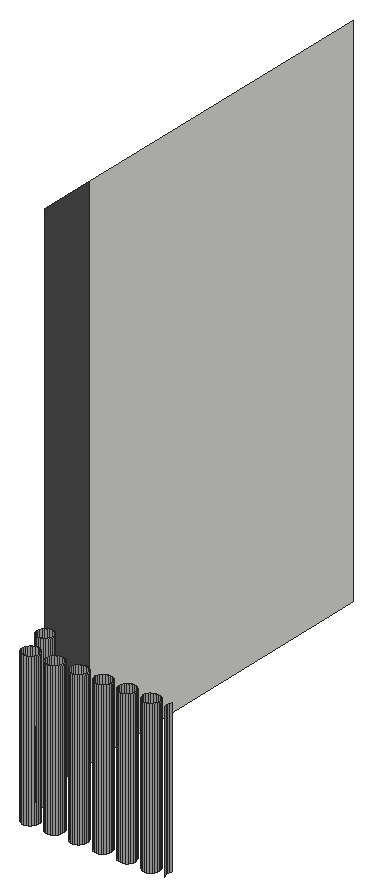
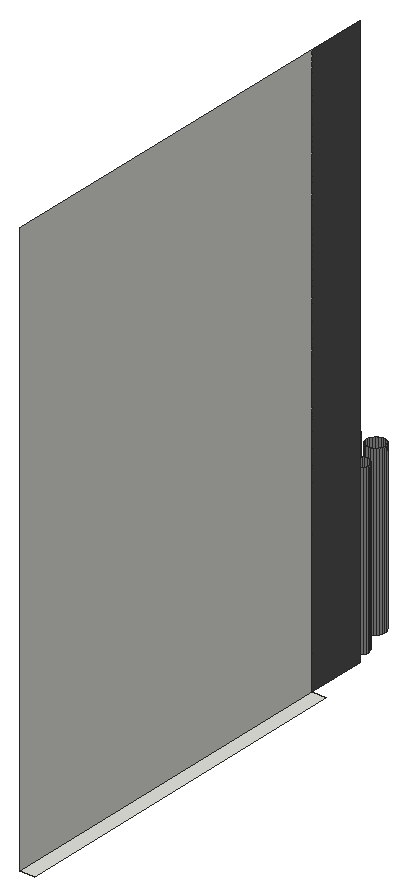
# SketchUp Ruby script. Lengths in inches.
U = 1.inch
M = Sketchup.active_model
def pt(a) = Geom::Point3d.new(a.map { |v| v * U })
def face(e, loops, mat)
  f = e.add_face(loops[0].map { |a| pt(a) })
  loops[1..].each { |l| e.add_face(l.map { |a| pt(a) }).erase! }
  f.material = f.back_material = mat if mat
  f
end
# faces: each face lists its corners as indices into pts; further lists are holes
def faces(e, pts, list, mat = nil) = list.each { |f| face(e, (f[0].is_a?(Array) ? f : [f]).map { |l| l.map { |i| pts[i] } }, mat) }
# xy, xz, yz: faces in a plane at the given z, y or x. An outline is a flat list of corners, or four numbers for a rectangle; further outlines are holes
def ring(l) = l.size == 4 ? [[l[0], l[1]], [l[2], l[1]], [l[2], l[3]], [l[0], l[3]]] : l.each_slice(2).to_a
def flat(e, list, mat, &to3) = list.each { |f| face(e, (f[0].is_a?(Array) ? f : [f]).map { |l| ring(l).map { |u, v| to3.(u, v) } }, mat) }
def xy(e, z, list, mat = nil) = flat(e, list, mat) { |x, y| [x, y, z] }
def xz(e, y, list, mat = nil) = flat(e, list, mat) { |x, z| [x, y, z] }
def yz(e, x, list, mat = nil) = flat(e, list, mat) { |y, z| [x, y, z] }
def lines(e, pts, list) = list.each { |a, b| e.add_line(pt(pts[a]), pt(pts[b])) }
# prism: a flat outline (further loops are holes) pulled along v
def prism(e, loops, v, mat = nil)
  f = face(e, loops, mat); d = Geom::Vector3d.new(v.map { |x| x * U })
  f.pushpull(f.normal.samedirection?(d) ? d.length : -d.length)
end
def box(e, o, s, mat = nil) = prism(e, [[o, [o[0] + s[0], o[1], o[2]], [o[0] + s[0], o[1] + s[1], o[2]], [o[0], o[1] + s[1], o[2]]]], [0, 0, s[2]], mat)
def at(x, y, z, deg = 0) = Geom::Transformation.translation(pt([x, y, z])) * Geom::Transformation.rotation(ORIGIN, Z_AXIS, deg.degrees)
def axes(o, x, y, z) = Geom::Transformation.new([*x, 0, *y, 0, *z, 0, *pt(o).to_a, 1])
def part(name) = M.definitions.add(name)
# library, detail: a bought-in or finely detailed component or shape, given as its bounding box
def library(name, o, s) = part(name).tap { |d| box(d.entities, o, s) }
def detail(e, o, s) = box(e.add_group.entities, o, s)
def put(e, d, t, mat = nil) = e.add_instance(d, t).tap { |i| i.material = mat if mat }
def group(e, t, mat = nil) = e.add_group.tap { |g| g.transformation = t; g.material = mat if mat }.entities
root = M.entities
M.materials.add("[0132_LightGray]").color = [169, 169, 169]
M.materials.add("[0135_DarkGray]").color = [81, 81, 81]
xy(root,638.72,[[254.33,31.93,253.97,31.97,253.64,32.11,253.36,32.33,253.14,32.62,253,32.95,252.95,33.3,253,33.66,253.14,33.99,253.36,34.28,253.64,34.49,253.97,34.63,254.33,34.68,254.68,34.63,255.02,34.49,255.3,34.28,255.52,33.99,255.66,33.66,255.7,33.3,255.66,32.95,255.52,32.62,255.3,32.33,255.02,32.11,254.68,31.97],[258.33,31.93,257.97,31.97,257.64,32.11,257.36,32.33,257.14,32.62,257,32.95,256.95,33.3,257,33.66,257.14,33.99,257.36,34.28,257.64,34.49,257.97,34.63,258.33,34.68,258.68,34.63,259.02,34.49,259.3,34.28,259.52,33.99,259.66,33.66,259.7,33.3,259.66,32.95,259.52,32.62,259.3,32.33,259.02,32.11,258.68,31.97],[262.33,31.93,261.97,31.97,261.64,32.11,261.36,32.33,261.14,32.62,261,32.95,260.95,33.3,261,33.66,261.14,33.99,261.36,34.28,261.64,34.49,261.97,34.63,262.33,34.68,262.68,34.63,263.02,34.49,263.3,34.28,263.52,33.99,263.66,33.66,263.7,33.3,263.66,32.95,263.52,32.62,263.3,32.33,263.02,32.11,262.68,31.97],[266.33,31.93,265.97,31.97,265.64,32.11,265.36,32.33,265.14,32.62,265,32.95,264.95,33.3,265,33.66,265.14,33.99,265.36,34.28,265.64,34.49,265.97,34.63,266.33,34.68,266.68,34.63,267.02,34.49,267.3,34.28,267.52,33.99,267.66,33.66,267.7,33.3,267.66,32.95,267.52,32.62,267.3,32.33,267.02,32.11,266.68,31.97],[244.88,36.8,244.54,36.84,244.22,36.97,243.95,37.18,243.74,37.45,243.61,37.77,243.57,38.11,243.61,38.45,243.74,38.77,243.95,39.04,244.22,39.25,244.54,39.38,244.88,39.42,245.22,39.38,245.53,39.25,245.81,39.04,246.01,38.77,246.15,38.45,246.19,38.11,246.15,37.77,246.01,37.45,245.81,37.18,245.53,36.97,245.22,36.84],
  [240.7,49.6875,242.82,104.375]])
yz(root,242.82,[[49.6875,638.72,104.375,725.13]])
yz(root,242.82,[[40.6875,638.72,49.6875,725.13]],"[0135_DarkGray]")
p = [[245.97,31.97,638.72],[246.33,31.93,638.72],[246.33,31.93,663.85],[245.97,31.97,663.85],[246.68,31.97,638.72],[246.68,31.97,663.85],
  [249.97,31.97,638.72],[250.33,31.93,638.72],[250.33,31.93,663.85],[249.97,31.97,663.85],[250.68,31.97,638.72],[250.68,31.97,663.85],
  [253.97,31.97,638.72],[254.33,31.93,638.72],[254.33,31.93,663.85],[253.97,31.97,663.85],[254.68,31.97,638.72],[254.68,31.97,663.85],
  [257.97,31.97,638.72],[258.33,31.93,638.72],[258.33,31.93,663.85],[257.97,31.97,663.85],[258.68,31.97,638.72],[258.68,31.97,663.85],
  [261.97,31.97,638.72],[262.33,31.93,638.72],[262.33,31.93,663.85],[261.97,31.97,663.85],[262.68,31.97,638.72],[262.68,31.97,663.85],
  [265.97,31.97,638.72],[266.33,31.93,638.72],[266.33,31.93,663.85],[265.97,31.97,663.85],[266.68,31.97,638.72],[266.68,31.97,663.85],
  [245.64,32.11,638.72],[245.64,32.11,663.85],[247.02,32.11,638.72],[247.02,32.11,663.85],[249.64,32.11,638.72],[249.64,32.11,663.85],
  [251.02,32.11,638.72],[251.02,32.11,663.85],[253.64,32.11,638.72],[253.64,32.11,663.85],[255.02,32.11,638.72],[255.02,32.11,663.85],
  [257.64,32.11,638.72],[257.64,32.11,663.85],[259.02,32.11,638.72],[259.02,32.11,663.85],[261.64,32.11,638.72],[261.64,32.11,663.85],
  [263.02,32.11,638.72],[263.02,32.11,663.85],[265.64,32.11,638.72],[265.64,32.11,663.85],[267.02,32.11,638.72],[267.02,32.11,663.85],
  [245.36,32.33,638.72],[245.36,32.33,663.85],[247.3,32.33,638.72],[247.3,32.33,663.85],[249.36,32.33,638.72],[249.36,32.33,663.85],
  [251.3,32.33,638.72],[251.3,32.33,663.85],[253.36,32.33,638.72],[253.36,32.33,663.85],[255.3,32.33,638.72],[255.3,32.33,663.85],
  [257.36,32.33,638.72],[257.36,32.33,663.85],[259.3,32.33,638.72],[259.3,32.33,663.85],[261.36,32.33,638.72],[261.36,32.33,663.85],
  [263.3,32.33,638.72],[263.3,32.33,663.85],[265.36,32.33,638.72],[265.36,32.33,663.85],[267.3,32.33,638.72],[267.3,32.33,663.85],
  [245.14,32.62,638.72],[245.14,32.62,663.85],[247.52,32.62,638.72],[247.52,32.62,663.85],[249.14,32.62,638.72],[249.14,32.62,663.85],
  [251.52,32.62,638.72],[251.52,32.62,663.85],[253.14,32.62,638.72],[253.14,32.62,663.85],[255.52,32.62,638.72],[255.52,32.62,663.85],
  [257.14,32.62,638.72],[257.14,32.62,663.85],[259.52,32.62,638.72],[259.52,32.62,663.85],[261.14,32.62,638.72],[261.14,32.62,663.85],
  [263.52,32.62,638.72],[263.52,32.62,663.85],[265.14,32.62,638.72],[265.14,32.62,663.85],[267.52,32.62,638.72],[267.52,32.62,663.85],
  [245,32.95,638.72],[245,32.95,663.85],[247.66,32.95,638.72],[247.66,32.95,663.85],[249,32.95,638.72],[249,32.95,663.85],
  [251.66,32.95,638.72],[251.66,32.95,663.85],[253,32.95,638.72],[253,32.95,663.85],[255.66,32.95,638.72],[255.66,32.95,663.85],
  [257,32.95,638.72],[257,32.95,663.85],[259.66,32.95,638.72],[259.66,32.95,663.85],[261,32.95,638.72],[261,32.95,663.85],
  [263.66,32.95,638.72],[263.66,32.95,663.85],[265,32.95,638.72],[265,32.95,663.85],[267.66,32.95,638.72],[267.66,32.95,663.85],
  [269,32.95,638.72],[269.14,32.62,638.72],[269.14,32.62,663.85],[269,32.95,663.85],[244.95,33.3,638.72],[244.95,33.3,663.85],
  [247.7,33.3,638.72],[247.7,33.3,663.85],[248.95,33.3,638.72],[248.95,33.3,663.85],[251.7,33.3,638.72],[251.7,33.3,663.85],
  [252.95,33.3,638.72],[252.95,33.3,663.85],[255.7,33.3,638.72],[255.7,33.3,663.85],[256.95,33.3,638.72],[256.95,33.3,663.85],
  [259.7,33.3,638.72],[259.7,33.3,663.85],[260.95,33.3,638.72],[260.95,33.3,663.85],[263.7,33.3,638.72],[263.7,33.3,663.85],
  [264.95,33.3,638.72],[264.95,33.3,663.85],[267.7,33.3,638.72],[267.7,33.3,663.85],[268.95,33.3,638.72],[268.95,33.3,663.85],
  [245,33.66,638.72],[245,33.66,663.85],[247.66,33.66,638.72],[247.66,33.66,663.85],[249,33.66,638.72],[249,33.66,663.85],
  [251.66,33.66,638.72],[251.66,33.66,663.85],[253,33.66,638.72],[253,33.66,663.85],[255.66,33.66,638.72],[255.66,33.66,663.85],
  [257,33.66,638.72],[257,33.66,663.85],[259.66,33.66,638.72],[259.66,33.66,663.85],[261,33.66,638.72],[261,33.66,663.85],
  [263.66,33.66,638.72],[263.66,33.66,663.85],[265,33.66,638.72],[265,33.66,663.85],[267.66,33.66,638.72],[267.66,33.66,663.85],
  [269,33.66,638.72],[269,33.66,663.85],[245.14,33.99,638.72],[245.14,33.99,663.85],[247.52,33.99,638.72],[247.52,33.99,663.85],
  [249.14,33.99,638.72],[249.14,33.99,663.85],[251.52,33.99,638.72],[251.52,33.99,663.85],[253.14,33.99,638.72],[253.14,33.99,663.85],
  [255.52,33.99,638.72],[255.52,33.99,663.85],[257.14,33.99,638.72],[257.14,33.99,663.85],[259.52,33.99,638.72],[259.52,33.99,663.85],
  [261.14,33.99,638.72],[261.14,33.99,663.85],[263.52,33.99,638.72],[263.52,33.99,663.85],[265.14,33.99,638.72],[265.14,33.99,663.85],
  [267.52,33.99,638.72],[267.52,33.99,663.85],[269.14,33.99,638.72],[269.14,33.99,663.85],[245.36,34.28,638.72],[245.36,34.28,663.85],
  [247.3,34.28,638.72],[247.3,34.28,663.85],[249.36,34.28,638.72],[249.36,34.28,663.85],[251.3,34.28,638.72],[251.3,34.28,663.85],
  [253.36,34.28,638.72],[253.36,34.28,663.85],[255.3,34.28,638.72],[255.3,34.28,663.85],[257.36,34.28,638.72],[257.36,34.28,663.85],
  [259.3,34.28,638.72],[259.3,34.28,663.85],[261.36,34.28,638.72],[261.36,34.28,663.85],[263.3,34.28,638.72],[263.3,34.28,663.85],
  [265.36,34.28,638.72],[265.36,34.28,663.85],[267.3,34.28,638.72],[267.3,34.28,663.85],[245.64,34.49,638.72],[245.64,34.49,663.85],
  [247.02,34.49,638.72],[247.02,34.49,663.85],[249.64,34.49,638.72],[249.64,34.49,663.85],[251.02,34.49,638.72],[251.02,34.49,663.85],
  [253.64,34.49,638.72],[253.64,34.49,663.85],[255.02,34.49,638.72],[255.02,34.49,663.85],[257.64,34.49,638.72],[257.64,34.49,663.85],
  [259.02,34.49,638.72],[259.02,34.49,663.85],[261.64,34.49,638.72],[261.64,34.49,663.85],[263.02,34.49,638.72],[263.02,34.49,663.85],
  [265.64,34.49,638.72],[265.64,34.49,663.85],[267.02,34.49,638.72],[267.02,34.49,663.85],[245.97,34.63,638.72],[245.97,34.63,663.85],
  [246.68,34.63,638.72],[246.68,34.63,663.85],[249.97,34.63,638.72],[249.97,34.63,663.85],[250.68,34.63,638.72],[250.68,34.63,663.85],
  [253.97,34.63,638.72],[253.97,34.63,663.85],[254.68,34.63,638.72],[254.68,34.63,663.85],[257.97,34.63,638.72],[257.97,34.63,663.85],
  [258.68,34.63,638.72],[258.68,34.63,663.85],[261.97,34.63,638.72],[261.97,34.63,663.85],[262.68,34.63,638.72],[262.68,34.63,663.85],
  [265.97,34.63,638.72],[265.97,34.63,663.85],[266.68,34.63,638.72],[266.68,34.63,663.85],[246.33,34.68,638.72],[246.33,34.68,663.85],
  [250.33,34.68,638.72],[250.33,34.68,663.85],[254.33,34.68,638.72],[254.33,34.68,663.85],[258.33,34.68,638.72],[258.33,34.68,663.85],
  [262.33,34.68,638.72],[262.33,34.68,663.85],[266.33,34.68,638.72],[266.33,34.68,663.85],[244.22,36.97,638.72],[244.54,36.84,638.72],
  [244.54,36.84,663.85],[244.22,36.97,663.85],[244.88,36.8,638.72],[244.88,36.8,663.85],[245.22,36.84,638.72],[245.22,36.84,663.85],
  [245.53,36.97,638.72],[245.53,36.97,663.85],[243.95,37.18,638.72],[243.95,37.18,663.85],[245.81,37.18,638.72],[245.81,37.18,663.85],
  [243.74,37.45,638.72],[243.74,37.45,663.85],[246.01,37.45,638.72],[246.01,37.45,663.85],[243.61,37.77,638.72],[243.61,37.77,663.85],
  [246.15,37.77,638.72],[246.15,37.77,663.85],[243.57,38.11,638.72],[243.57,38.11,663.85],[246.19,38.11,638.72],[246.19,38.11,663.85],
  [243.61,38.45,638.72],[243.61,38.45,663.85],[246.15,38.45,638.72],[246.15,38.45,663.85],[243.74,38.77,638.72],[243.74,38.77,663.85],
  [246.01,38.77,638.72],[246.01,38.77,663.85],[243.95,39.04,638.72],[243.95,39.04,663.85],[245.81,39.04,638.72],[245.81,39.04,663.85],
  [244.22,39.25,638.72],[244.22,39.25,663.85],[245.53,39.25,638.72],[245.53,39.25,663.85],[244.54,39.38,638.72],[244.54,39.38,663.85],
  [245.22,39.38,638.72],[245.22,39.38,663.85],[244.88,39.42,638.72],[244.88,39.42,663.85]]
faces(root,p,[[0,1,2,3],[1,4,5,2],[6,7,8,9],[7,10,11,8],[12,13,14,15],[13,16,17,14],[18,19,20,21],[19,22,23,20],
  [24,25,26,27],[25,28,29,26],[30,31,32,33],[31,34,35,32],[36,0,3,37],[4,38,39,5],[40,6,9,41],[10,42,43,11],
  [44,12,15,45],[16,46,47,17],[48,18,21,49],[22,50,51,23],[52,24,27,53],[28,54,55,29],[56,30,33,57],[34,58,59,35],
  [60,36,37,61],[38,62,63,39],[64,40,41,65],[42,66,67,43],[68,44,45,69],[46,70,71,47],[72,48,49,73],[50,74,75,51],
  [76,52,53,77],[54,78,79,55],[80,56,57,81],[58,82,83,59],[84,60,61,85],[62,86,87,63],[88,64,65,89],[66,90,91,67],
  [92,68,69,93],[70,94,95,71],[96,72,73,97],[74,98,99,75],[100,76,77,101],[78,102,103,79],[104,80,81,105],[82,106,107,83],
  [108,84,85,109],[86,110,111,87],[112,88,89,113],[90,114,115,91],[116,92,93,117],[94,118,119,95],[120,96,97,121],[98,122,123,99],
  [124,100,101,125],[102,126,127,103],[128,104,105,129],[106,130,131,107],[132,133,134,135],[136,108,109,137],[110,138,139,111],[140,112,113,141],
  [114,142,143,115],[144,116,117,145],[118,146,147,119],[148,120,121,149],[122,150,151,123],[152,124,125,153],[126,154,155,127],[156,128,129,157],
  [130,158,159,131],[160,132,135,161],[162,136,137,163],[138,164,165,139],[166,140,141,167],[142,168,169,143],[170,144,145,171],[146,172,173,147],
  [174,148,149,175],[150,176,177,151],[178,152,153,179],[154,180,181,155],[182,156,157,183],[158,184,185,159],[186,160,161,187],[188,162,163,189],
  [164,190,191,165],[192,166,167,193],[168,194,195,169],[196,170,171,197],[172,198,199,173],[200,174,175,201],[176,202,203,177],[204,178,179,205],
  [180,206,207,181],[208,182,183,209],[184,210,211,185],[212,186,187,213],[214,188,189,215],[190,216,217,191],[218,192,193,219],[194,220,221,195],
  [222,196,197,223],[198,224,225,199],[226,200,201,227],[202,228,229,203],[230,204,205,231],[206,232,233,207],[234,208,209,235],[210,236,237,211],
  [238,214,215,239],[216,240,241,217],[242,218,219,243],[220,244,245,221],[246,222,223,247],[224,248,249,225],[250,226,227,251],[228,252,253,229],
  [254,230,231,255],[232,256,257,233],[258,234,235,259],[236,260,261,237],[262,238,239,263],[240,264,265,241],[266,242,243,267],[244,268,269,245],
  [270,246,247,271],[248,272,273,249],[274,250,251,275],[252,276,277,253],[278,254,255,279],[256,280,281,257],[282,258,259,283],[260,284,285,261],
  [286,262,263,287],[264,286,287,265],[288,266,267,289],[268,288,289,269],[290,270,271,291],[272,290,291,273],[292,274,275,293],[276,292,293,277],
  [294,278,279,295],[280,294,295,281],[296,282,283,297],[284,296,297,285],[298,299,300,301],[299,302,303,300],[302,304,305,303],[304,306,307,305],
  [308,298,301,309],[306,310,311,307],[312,308,309,313],[310,314,315,311],[316,312,313,317],[314,318,319,315],[320,316,317,321],[318,322,323,319],
  [324,320,321,325],[322,326,327,323],[328,324,325,329],[326,330,331,327],[332,328,329,333],[330,334,335,331],[336,332,333,337],[334,338,339,335],
  [340,336,337,341],[338,342,343,339],[344,340,341,345],[342,344,345,343]],"[0132_LightGray]")
